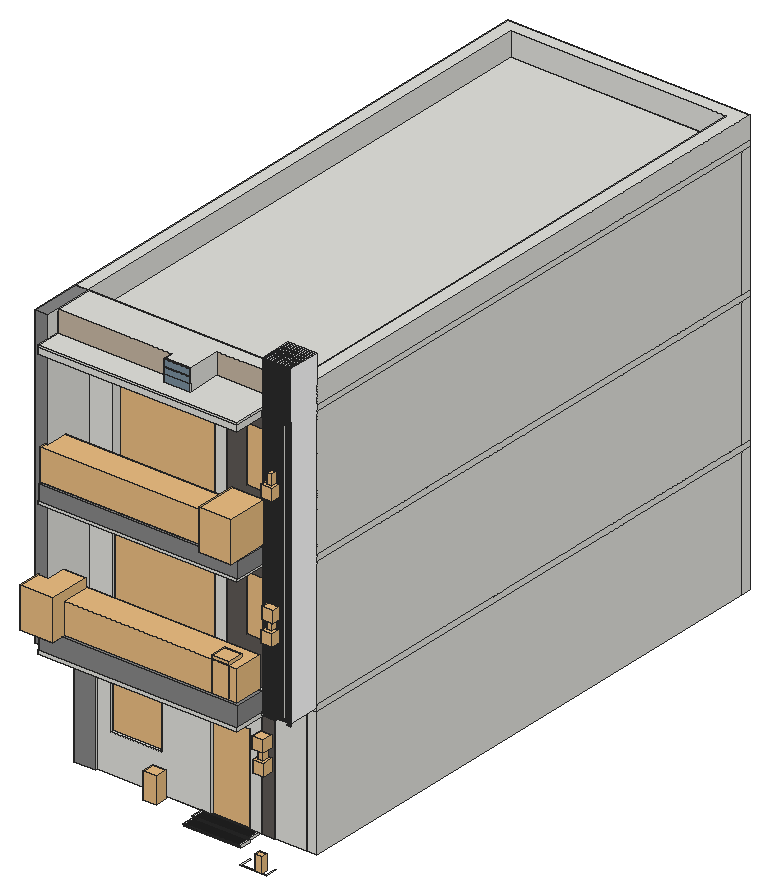
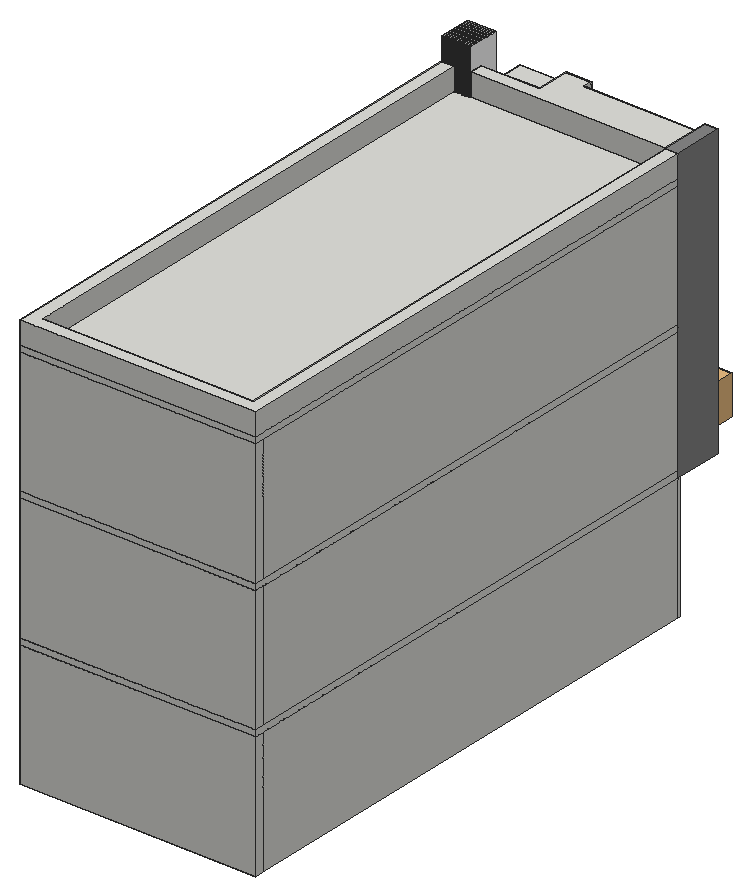
# SketchUp Ruby script. Lengths in inches.
U = 1.inch
M = Sketchup.active_model
def pt(a) = Geom::Point3d.new(a.map { |v| v * U })
def face(e, loops, mat)
  f = e.add_face(loops[0].map { |a| pt(a) })
  loops[1..].each { |l| e.add_face(l.map { |a| pt(a) }).erase! }
  f.material = f.back_material = mat if mat
  f
end
# faces: each face lists its corners as indices into pts; further lists are holes
def faces(e, pts, list, mat = nil) = list.each { |f| face(e, (f[0].is_a?(Array) ? f : [f]).map { |l| l.map { |i| pts[i] } }, mat) }
# xy, xz, yz: faces in a plane at the given z, y or x. An outline is a flat list of corners, or four numbers for a rectangle; further outlines are holes
def ring(l) = l.size == 4 ? [[l[0], l[1]], [l[2], l[1]], [l[2], l[3]], [l[0], l[3]]] : l.each_slice(2).to_a
def flat(e, list, mat, &to3) = list.each { |f| face(e, (f[0].is_a?(Array) ? f : [f]).map { |l| ring(l).map { |u, v| to3.(u, v) } }, mat) }
def xy(e, z, list, mat = nil) = flat(e, list, mat) { |x, y| [x, y, z] }
def xz(e, y, list, mat = nil) = flat(e, list, mat) { |x, z| [x, y, z] }
def yz(e, x, list, mat = nil) = flat(e, list, mat) { |y, z| [x, y, z] }
def lines(e, pts, list) = list.each { |a, b| e.add_line(pt(pts[a]), pt(pts[b])) }
# prism: a flat outline (further loops are holes) pulled along v
def prism(e, loops, v, mat = nil)
  f = face(e, loops, mat); d = Geom::Vector3d.new(v.map { |x| x * U })
  f.pushpull(f.normal.samedirection?(d) ? d.length : -d.length)
end
def box(e, o, s, mat = nil) = prism(e, [[o, [o[0] + s[0], o[1], o[2]], [o[0] + s[0], o[1] + s[1], o[2]], [o[0], o[1] + s[1], o[2]]]], [0, 0, s[2]], mat)
def at(x, y, z, deg = 0) = Geom::Transformation.translation(pt([x, y, z])) * Geom::Transformation.rotation(ORIGIN, Z_AXIS, deg.degrees)
def axes(o, x, y, z) = Geom::Transformation.new([*x, 0, *y, 0, *z, 0, *pt(o).to_a, 1])
def part(name) = M.definitions.add(name)
# library, detail: a bought-in or finely detailed component or shape, given as its bounding box
def library(name, o, s) = part(name).tap { |d| box(d.entities, o, s) }
def detail(e, o, s) = box(e.add_group.entities, o, s)
def put(e, d, t, mat = nil) = e.add_instance(d, t).tap { |i| i.material = mat if mat }
def group(e, t, mat = nil) = e.add_group.tap { |g| g.transformation = t; g.material = mat if mat }.entities
root = M.entities
M.materials.add("Bricks A03 100cm").color = [95, 90, 86]
M.materials.add("Marble White 602 38.29cm").color = [255, 255, 255]
M.materials.add("Pearl Cream 2cm").color = [199, 183, 163]
M.materials.add("Tiles Marble Black 01 160cm").color = [32, 32, 32]
M.materials.add("Wall Paint Bumpy 01 Gray 100cm").color = [135, 135, 135]
M.materials.add("Wall Paint Dusk Blue Satin 300cm").color = [122, 143, 157]
M.materials.add("Wood Amboyan 13.2cm").color = [255, 255, 255]
M.materials.add("Wood Teak 33-35 100cm").color = [135, 81, 33]
c1 = library("Potted Plant 13",[-10,-7.28,0],[18.93,15.17,39.22])
c2 = part("Component\#12")
xy(c2.entities,0,[[0,0,53.8125,10.8125]])
xy(c2.entities,1.8125,[[0,-0.5,2,0],[2,-0.5,51.8125,0],[51.8125,-0.5,53.8125,0]])
xy(c2.entities,2.125,[[51.8125,-0.5,53.8125,10.8125]])
xy(c2.entities,2.125,[[0,-0.5,2,10.8125]],"Marble White 602 38.29cm")
xy(c2.entities,2.125,[[2,-0.5,51.8125,10.8125]],"Tiles Marble Black 01 160cm")
xz(c2.entities,-0.5,[[0,1.8125,53.8125,2.125]],"Marble White 602 38.29cm")
xz(c2.entities,0,[[0,0,53.8125,1.8125]],"Tiles Marble Black 01 160cm")
xz(c2.entities,10.8125,[[0,0,53.8125,2.125]])
yz(c2.entities,0,[[0,0,0,1.8125,-0.5,1.8125,-0.5,2.125,10.8125,2.125,10.8125,0]])
yz(c2.entities,53.8125,[[0,0,10.8125,0,10.8125,2.125,-0.5,2.125,-0.5,1.8125,0,1.8125]])
c3 = library("Indoor Plant 004",[-26.75,-21.09,0],[44.44,41.03,87.36])
c4 = library("Door 243 065",[-19.36,-2.49,0],[38.72,4.98,81.96])
c5 = part("Group\#2")
box(c5.entities,[0,0,0],[226.5,9,120])
c6 = part("Group\#5")
xy(c6.entities,0,[[0,0,72,4.5],[102,0,102,4.5,108,4.5,108,124.5,112.5,124.5,112.5,4.5,118.5,4.5,118.5,0],[148.5,0,208.5,4.5]])
xy(c6.entities,84,[[72,0,102,4.5],[118.5,0,148.5,4.5]])
xy(c6.entities,120,[[0,0,208.5,0,208.5,4.5,112.5,4.5,112.5,124.5,108,124.5,108,4.5,0,4.5]])
xz(c6.entities,0,[[0,0,72,0,72,84,102,84,102,0,118.5,0,118.5,84,148.5,84,148.5,0,208.5,0,208.5,120,0,120]])
xz(c6.entities,4.5,[[0,0,0,120,108,120,108,0,102,0,102,84,72,84,72,0],[112.5,0,112.5,120,208.5,120,208.5,0,148.5,0,148.5,84,118.5,84,118.5,0]])
xz(c6.entities,124.5,[[108,0,112.5,120]])
yz(c6.entities,0,[[0,0,4.5,120]])
yz(c6.entities,72,[[0,0,4.5,84]])
yz(c6.entities,102,[[0,0,4.5,84]])
yz(c6.entities,108,[[4.5,0,124.5,120]])
yz(c6.entities,112.5,[[4.5,0,124.5,120]])
yz(c6.entities,118.5,[[0,0,4.5,84]])
yz(c6.entities,148.5,[[0,0,4.5,84]])
yz(c6.entities,208.5,[[0,0,4.5,120]])
c7 = part("Group\#4")
box(c7.entities,[0,0,0],[9,498,120])
c8 = library("Window 109 011",[-27.22,-3.26,-0.09],[54.45,6.58,70.7])
c9 = library("Spot Light\#2",[-5.1,-5.1,-11.05],[10.2,10.2,11.05])
c10 = library("Lamp Wall Outdoor 94-02",[-1.89,-4.65,-3.17],[3.78,4.65,6.35])
c11 = library("Spot Light\#1",[-5.1,-5.1,-11.05],[10.2,10.2,11.05])
c12 = library("Sphere Light\#10",[-3,-3,-3],[6,6,6])
c13 = library("Sphere Light\#9",[-3,-3,-3],[6,6,6])
c14 = library("Sphere Light\#12",[-3,-3,-3],[6,6,6])
c15 = library("Sphere Light\#11",[-3,-3,-3],[6,6,6])
c16 = part("Vertical panel")
box(c16.entities,[0,0,-125.125],[0.9,30,298.0625],"Wood Amboyan 13.2cm")
c17 = library("Climbing Plant 21-17",[-12.91,-12.55,0],[25.47,24.76,31.08])
c18 = part("Group\#11")
g1 = group(c18.entities,at(9,9,0))
prism(g1,[[[0,172.5,0],[142.89,172.5,0],[142.89,0,0],[138.39,0,0],[138.39,168.03,0],[0,168.03,0]]],[0,0,120])
g2 = group(c18.entities,at(9,0,0))
prism(g2,[[[208.5,9,0],[0,9,0],[0,9,120],[208.5,9,120]],[[26.125,9,96],[26.125,9,12],[122.125,9,12],[122.125,9,96]]],[0,-9,0])
put(c18.entities,c7,at(0,0,0))
put(c18.entities,c6,at(9,373.5,0))
g3 = group(c18.entities,at(217.5,0,0))
box(g3,[0,0,0],[9,498,120])
c19 = library("Window 46-47",[-61.02,-2.17,0],[122.04,4.34,74.02])
c20 = library("Group\#21",[0,0,0],[183.84,26.65,37.57])
c21 = library("Potted Plant 02",[-16.98,-19.78,0],[30.04,38.68,37.52])
c22 = library("Sphere Light\#5",[-3,-3,-3],[6,6,6])
c23 = library("Sphere Light\#6",[-3,-3,-3],[6,6,6])
c24 = library("Sphere Light\#7",[-3,-3,-3],[6,6,6])
c25 = library("Sphere Light\#8",[-3,-3,-3],[6,6,6])
c26 = library("Spot Light",[-5.1,-5.1,-11.05],[10.2,10.2,11.05])
c27 = library("Sphere Light",[-3,-3,-3],[6,6,6])
c28 = library("Sphere Light\#2",[-3,-3,-3],[6,6,6])
c29 = library("Sphere Light\#3",[-3,-3,-3],[6,6,6])
c30 = library("Sphere Light\#4",[-3,-3,-3],[6,6,6])
xy(root,-3.9,[[462.69,202.57,487.92,202.57,487.92,213.79,486.92,213.79,486.92,203.57,463.69,203.57,463.69,214.57,462.69,214.57]])
xy(root,0,[[450.69,243.57,462.69,244.57]])
xy(root,120,[[275.19,196.58,287.94,244.57],[450.69,243.57,462.69,244.57]])
xy(root,121.5,[[474.63,213.79,487.92,214.57],[497.86,213.79,501.69,214.57]])
xy(root,123.3125,[[475.6,214.57,476.76,244.57]])
xy(root,125.96,[[474.63,213.79,495.69,214.57]])
xy(root,248.4375,[[287.94,185.57,474.63,196.57],[462.63,196.57,474.63,214.57]],"Wall Paint Bumpy 01 Gray 100cm")
xy(root,262.3,[[287.94,185.57,474.63,185.57,474.63,214.57,468.63,214.57,468.63,191.07,287.94,191.07],[287.94,191.07,468.63,191.07,468.63,214.57,462.63,214.57,462.63,196.57,287.94,196.57]],"Wall Paint Bumpy 01 Gray 100cm")
xy(root,372,[[474.63,213.79,495.69,214.57]])
xy(root,378,[[287.94,184.57,474.63,200.14],[287.94,200.14,474.63,244.57],[474.63,213.79,501.69,214.57],[275.19,244.57,275.19,751.57,501.69,751.57,501.69,244.57,489.69,244.57,489.69,739.57,287.19,739.57,287.19,244.57]])
xy(root,379.5625,[[287.94,184.57,474.63,184.57,474.63,231.57,418.69,231.57,418.69,199.14,394.69,199.14,394.69,208.45,287.94,208.45],[394.69,199.14,418.69,200.14]])
xy(root,386.21,[[394.69,199.14,418.69,200.14]])
xy(root,386.52,[[394.69,199.14,418.69,200.14]])
xy(root,392.85,[[394.69,199.14,418.69,200.14]])
xy(root,393.17,[[394.69,199.14,418.69,200.14]])
xy(root,399.5,[[394.69,199.14,418.69,200.14],[394.69,200.14,418.69,200.14,418.69,231.57,474.63,231.57,474.63,244.57,287.94,244.57,287.94,208.45,394.69,208.45],[275.19,244.57,287.19,244.57,287.19,739.57,489.69,739.57,489.69,244.57,501.69,244.57,501.69,751.57,275.19,751.57]])
xy(root,399.5,[[275.19,196.58,287.94,244.57]],"Wall Paint Bumpy 01 Gray 100cm")
xz(root,184.57,[[287.94,378,474.63,379.5625]])
xz(root,185.57,[[287.94,248.4375,474.63,262.3]],"Wall Paint Bumpy 01 Gray 100cm")
xz(root,196.57,[[287.94,248.4375,462.63,262.3]],"Wall Paint Bumpy 01 Gray 100cm")
xz(root,196.58,[[275.19,120,287.94,399.5]],"Wall Paint Bumpy 01 Gray 100cm")
xz(root,199.14,[[394.69,379.5625,418.69,386.21],[394.69,386.52,418.69,392.85],[394.69,393.17,418.69,399.5]],"Wall Paint Dusk Blue Satin 300cm")
xz(root,200.14,[[394.69,379.5625,418.69,386.21],[394.69,386.21,418.69,386.52],[394.69,386.52,418.69,392.85],[394.69,392.85,418.69,393.17],[394.69,393.17,418.69,399.5]])
xz(root,208.45,[[287.94,379.5625,394.69,399.5]],"Pearl Cream 2cm")
xz(root,214.57,[[475.6,121.5,476.76,123.3125]])
xz(root,214.57,[[462.63,248.4375,474.63,262.3]],"Wall Paint Bumpy 01 Gray 100cm")
xz(root,231.57,[[418.69,379.5625,474.63,399.5]],"Pearl Cream 2cm")
xz(root,243.57,[[450.69,0,462.69,120]],"Bricks A03 100cm")
xz(root,244.57,[[450.69,0,462.69,120],[275.19,120,275.19,378,287.19,378,287.19,399.5,287.94,399.5,287.94,120],[275.19,378,287.19,399.5],[287.94,378,474.63,399.5],[489.69,378,501.69,399.5]])
xz(root,739.57,[[287.19,378,489.69,399.5]])
xz(root,751.57,[[275.19,378,501.69,399.5]])
yz(root,275.19,[[244.57,378,751.57,399.5]])
yz(root,275.19,[[196.58,120,244.57,399.5]],"Wall Paint Bumpy 01 Gray 100cm")
yz(root,287.19,[[244.57,378,739.57,399.5]])
yz(root,287.94,[[196.58,120,244.57,378],[184.57,378,196.58,379.5625],[196.58,378,200.14,379.5625],[200.14,378,244.57,378,244.57,399.5,208.45,399.5,208.45,379.5625,200.14,379.5625],[196.58,379.5625,208.45,399.5]])
yz(root,287.94,[[185.57,248.4375,196.57,262.3]],"Wall Paint Bumpy 01 Gray 100cm")
yz(root,394.69,[[199.14,379.5625,200.14,386.21],[200.14,379.5625,208.45,399.5],[199.14,386.52,200.14,392.85],[199.14,393.17,200.14,399.5]])
yz(root,418.69,[[199.14,379.5625,200.14,386.21],[200.14,379.5625,231.57,399.5],[199.14,386.52,200.14,392.85],[199.14,393.17,200.14,399.5]])
yz(root,450.69,[[243.57,0,244.57,120]],"Bricks A03 100cm")
yz(root,462.63,[[196.57,248.4375,214.57,262.3]],"Wall Paint Bumpy 01 Gray 100cm")
yz(root,462.69,[[243.57,0,244.57,120]])
yz(root,474.63,[[213.79,121.5,214.57,125.96],[213.79,372,214.57,378],[184.57,378,200.14,379.5625],[200.14,378,244.57,378,244.57,399.5,231.57,399.5,231.57,379.5625,200.14,379.5625]])
yz(root,474.63,[[185.57,248.4375,214.57,262.3]],"Wall Paint Bumpy 01 Gray 100cm")
yz(root,489.69,[[244.57,378,739.57,399.5]])
yz(root,495.69,[[213.79,125.96,214.57,372]])
yz(root,501.69,[[213.79,121.5,214.57,378],[244.57,378,751.57,399.5]])
put(root,c1,axes([480.23,205.93,-3.9],[0.36,0,0],[0,0.36,0],[0,0,0.36]))
put(root,c2,at(393.8,222.95,-3.75))
put(root,c2,at(393.8,233.76,-2.125))
put(root,c3,axes([358.04,235.82,-0.4375],[0.28,0,0],[0,0.28,0],[0,0,0.28]))
put(root,c4,axes([420.69,248.1,-0.07],[0.92977,0,0],[0,0.88,0],[0,0,1.02576]))
put(root,c5,at(275.19,742.57,0))
g4 = group(root,at(492.69,244.57,0))
box(g4,[0,0,0],[9,498,120])
put(root,c6,at(284.19,618.07,0))
g5 = group(root,at(284.19,253.57,0))
xy(g5,0,[[108,0,108,168,102,168,102,172.5,112.5,172.5,112.5,0],[0,168,66,172.5]])
xy(g5,84,[[66,168,102,172.5]])
xy(g5,120,[[108,0,112.5,0,112.5,172.5,0,172.5,0,168,108,168]])
xz(g5,0,[[108,0,112.5,120]])
xz(g5,168,[[0,0,66,0,66,84,102,84,102,0,108,0,108,120,0,120]])
xz(g5,172.5,[[0,0,0,120,112.5,120,112.5,0,102,0,102,84,66,84,66,0]])
yz(g5,0,[[168,0,172.5,120]])
yz(g5,66,[[168,0,172.5,84]])
yz(g5,102,[[168,0,172.5,84]])
yz(g5,108,[[0,0,168,120]])
yz(g5,112.5,[[0,0,172.5,120]])
g6 = group(root,at(275.19,244.57,0))
g7 = group(g6,at(0,0,0))
g8 = group(g7,at(9,0,0))
xy(g8,0,[[0,0,118.5,9],[154.5,0,208.5,9]])
xy(g8,36,[[24.5,0,72.5,9]])
xy(g8,84,[[24.5,0,72.5,9],[118.5,0,154.5,9]])
xy(g8,120,[[0,0,208.5,9]])
xz(g8,0,[[-9,0,0,120],[[0,0,118.5,0,118.5,84,154.5,84,154.5,0,208.5,0,208.5,120,0,120],[24.5,36,72.5,84]]])
xz(g8,9,[[[0,0,0,120,208.5,120,208.5,0,154.5,0,154.5,84,118.5,84,118.5,0],[24.5,36,72.5,84]]])
yz(g8,0,[[0,0,9,120]])
yz(g8,24.5,[[0,36,9,84]])
yz(g8,72.5,[[0,36,9,84]])
yz(g8,118.5,[[0,0,9,84]])
yz(g8,154.5,[[0,0,9,84]])
yz(g8,208.5,[[0,0,9,120]])
put(g7,c7,at(0,0,0))
g9 = group(g6,at(0,-2,0))
xy(g9,0,[[0,0,20.49,2]])
xy(g9,120,[[0,0,20.49,2]])
xz(g9,0,[[0,0,20.49,120]],"Wall Paint Bumpy 01 Gray 100cm")
xz(g9,2,[[0,0,20.49,120]])
yz(g9,0,[[0,0,2,120]])
yz(g9,20.49,[[0,0,2,120]])
put(root,c8,axes([332.69,247.98,36.06],[0.88154,0,0],[0,0.33,0],[0,0,0.67894]))
put(root,c9,at(477.13,211.42,86.71))
put(root,c10,axes([477.17,214.57,91.35],[1.15,0,0],[0,1.15,0],[0,0,1.472]))
put(root,c11,axes([476.56,211.54,95.12],[1,0,0],[0,1,0],[0,0,-1]))
put(root,c12,at(360.16,214.57,118))
put(root,c13,at(307.47,214.57,118))
put(root,c14,at(453.25,214.57,120))
put(root,c15,at(411.81,214.57,120))
g10 = group(root,at(275.19,244.57,120))
xy(g10,0,[[0,0,226.5,507]])
xy(g10,0,[[12.75,-60,199.4375,0]],"Wood Teak 33-35 100cm")
xy(g10,3.3125,[[12.75,-60,199.4375,-0.23]])
xy(g10,6,[[0,-0.23,199.4375,-0.23,199.4375,0,226.5,0,226.5,507,0,507]])
xz(g10,-60,[[12.75,0,199.4375,3.3125]])
xz(g10,-0.23,[[12.75,3.3125,199.4375,6]])
xz(g10,0,[[199.4375,0,226.5,6]])
xz(g10,507,[[0,0,226.5,6]])
yz(g10,0,[[0,0,-0.23,6,507,6,507,0]])
yz(g10,12.75,[[-60,0,-60,3.3125,-0.23,3.3125,-0.23,6,0,0]])
yz(g10,199.4375,[[-60,0,0,0,0,6,-0.23,6,-0.23,3.3125,-60,3.3125]])
yz(g10,226.5,[[0,0,507,6]])
p = [[0,-0.23,6],[0,0,0],[12.75,0,0],[12.75,-0.23,6]]
faces(g10,p,[[0,1,2,3]])
put(root,c1,at(388.95,203.24,123.3125))
put(root,c16,at(474.63,214.57,248.4375),"Wood Amboyan 13.2cm")
put(root,c16,at(476.34,214.57,248.4375))
put(root,c16,at(478.0625,214.57,248.4375))
put(root,c16,at(479.78,214.57,248.4375))
put(root,c16,at(481.49,214.57,248.4375))
put(root,c16,at(483.21,214.57,248.4375))
put(root,c16,at(484.93,214.57,248.4375))
put(root,c16,at(486.64,214.57,248.4375))
put(root,c16,at(488.36,214.57,248.4375))
put(root,c16,at(490.08,214.57,248.4375))
put(root,c16,at(491.79,214.57,248.4375))
put(root,c16,at(493.59,214.57,248.4375))
put(root,c16,at(495.39,214.57,248.4375))
put(root,c16,at(497.19,214.57,248.4375))
put(root,c16,at(498.99,214.57,248.4375))
put(root,c16,at(500.79,214.57,248.4375))
g11 = group(root,at(418.32,243.57,123.3125))
prism(g11,[[[0,1,0],[0,1,123.5625],[56.3125,1,123.5625],[56.3125,1,0]],[[18.16,1,92.6875],[18.16,1,39.75],[38.16,1,39.75],[38.16,1,92.6875]]],[0,-1,0],"Bricks A03 100cm")
g12 = group(root,at(287.94,184.57,123.3125))
xy(g12,0,[[0,1,0,12,174.6875,12,174.6875,30,186.6875,30,186.6875,1]],"Wall Paint Bumpy 01 Gray 100cm")
xy(g12,18,[[0,1,186.6875,1,186.6875,30,180.6875,30,180.6875,6.5,0,6.5],[0,6.5,180.6875,6.5,180.6875,30,174.6875,30,174.6875,12,0,12]],"Wall Paint Bumpy 01 Gray 100cm")
xz(g12,1,[[0,0,186.6875,18]],"Wall Paint Bumpy 01 Gray 100cm")
xz(g12,12,[[0,0,174.6875,18]],"Wall Paint Bumpy 01 Gray 100cm")
xz(g12,30,[[174.6875,0,186.6875,18]],"Wall Paint Bumpy 01 Gray 100cm")
yz(g12,0,[[1,0,12,18]],"Wall Paint Bumpy 01 Gray 100cm")
yz(g12,174.6875,[[12,0,30,18]],"Wall Paint Bumpy 01 Gray 100cm")
yz(g12,186.6875,[[1,0,30,18]],"Wall Paint Bumpy 01 Gray 100cm")
put(root,c17,axes([363.15,209.8,123.3125],[0.8505,0,0],[0,0.8505,0],[0,0,0.8505]))
g13 = group(root,at(275.19,244.57,126))
put(g13,c18,at(0,0,0))
put(g13,c5,at(0,498,0))
put(root,c19,axes([358.72,247.52,137.68],[0.78,0,0],[0,0.78,0],[0,0,1.13914]))
put(root,c3,axes([456.67,197.56,141.3125],[0.36,0,0],[0,0.36,0],[0,0,0.36]))
put(root,c20,axes([287.32,189.24,141.3125],[1,0,0],[0,1,0],[0,0,0.77]))
put(root,c21,at(295.92,195.1875,141.3125))
put(root,c8,axes([446.47,244.08,163.13],[0.36731,0,0],[0,-0.15202,0],[0,0,0.74878]))
put(root,c11,at(485.38,211.02,198.67))
put(root,c10,axes([485.37,214.57,203.3],[1.15,0,0],[0,1.15,0],[0,0,1.472]))
put(root,c11,axes([485.37,211.9375,207.07],[1,0,0],[0,1,0],[0,0,-1]))
put(root,c22,at(307.42,214.57,246))
put(root,c23,at(360.41,214.57,246))
put(root,c24,at(412.33,214.57,246))
put(root,c25,at(450.85,214.57,246))
g14 = group(root,at(275.19,244.57,246))
xy(g14,0,[[12.75,-60,12.75,0,0,0,0,507,226.5,507,226.5,0,199.4375,0,199.4375,-60]],"Wood Teak 33-35 100cm")
xy(g14,2.4375,[[12.75,-60,199.4375,0]])
xy(g14,6,[[0,0,226.5,507]])
xz(g14,-60,[[12.75,0,199.4375,2.4375]])
xz(g14,0,[[0,0,12.75,6],[199.4375,0,226.5,6],[12.75,2.4375,199.4375,6]])
xz(g14,507,[[0,0,226.5,6]])
yz(g14,0,[[0,0,507,6]])
yz(g14,12.75,[[-60,0,0,2.4375]])
yz(g14,199.4375,[[-60,0,0,2.4375]])
yz(g14,226.5,[[0,0,507,6]])
put(root,c3,axes([304.17,203.47,248.4375],[0.46,0,0],[0,0.46,0],[0,0,0.46]))
g15 = group(root,at(418.32,243.57,248.4375))
xy(g15,0,[[0,0,56.3125,1]])
xy(g15,39.75,[[18.16,0,38.16,1]])
xy(g15,92.6875,[[18.16,0,38.16,1]])
xy(g15,123.5625,[[0,0,56.3125,1]])
xz(g15,0,[[[0,0,56.3125,123.5625],[18.16,39.75,38.16,92.6875]]],"Bricks A03 100cm")
xz(g15,1,[[[0,0,56.3125,123.5625],[18.16,39.75,38.16,92.6875]]])
yz(g15,0,[[0,0,1,123.5625]],"Bricks A03 100cm")
yz(g15,18.16,[[0,39.75,1,92.6875]])
yz(g15,38.16,[[0,39.75,1,92.6875]])
yz(g15,56.3125,[[0,0,1,123.5625]])
put(root,c17,axes([393.67,207.85,248.4375],[0.74,0,0],[0,0.74,0],[0,0,0.74]))
g16 = group(root,at(275.19,244.57,252))
put(g16,c18,at(0,0,0))
put(g16,c5,at(0,498,0))
put(root,c20,axes([286.37,189.5,262.3],[1,0,0],[0,1,0],[0,0,0.77]))
put(root,c19,axes([358.27,253.01,263.5],[0.78726,0,0],[0,-0.25909,0],[0,0,1.13914]))
put(root,c21,at(462.63,196.57,264.68))
put(root,c8,axes([446.47,244.08,288.25],[0.36731,0,0],[0,-0.15202,0],[0,0,0.74878]))
put(root,c26,at(485.48,210.87,321.13))
put(root,c10,axes([485.37,214.57,325.77],[1.15,0,0],[0,1.15,0],[0,0,1.472]))
put(root,c27,at(307.3,214.57,372))
put(root,c28,at(450.84,214.57,372))
put(root,c29,at(412.3,214.57,372))
put(root,c30,at(360.22,214.57,372))
g17 = group(root,at(275.19,244.57,372))
xy(g17,0,[[12.75,-60,12.75,0,0,0,0,507,226.5,507,226.5,0,199.4375,0,199.4375,-60]],"Wood Teak 33-35 100cm")
xy(g17,6,[[12.75,-60,199.4375,-60,199.4375,0,226.5,0,226.5,507,0,507,0,0,12.75,0]])
xz(g17,-60,[[12.75,0,199.4375,6]])
xz(g17,0,[[0,0,12.75,6],[199.4375,0,226.5,6]])
xz(g17,507,[[0,0,226.5,6]])
yz(g17,0,[[0,0,507,6]])
yz(g17,12.75,[[-60,0,0,6]])
yz(g17,199.4375,[[-60,0,0,6]])
yz(g17,226.5,[[0,0,507,6]])
